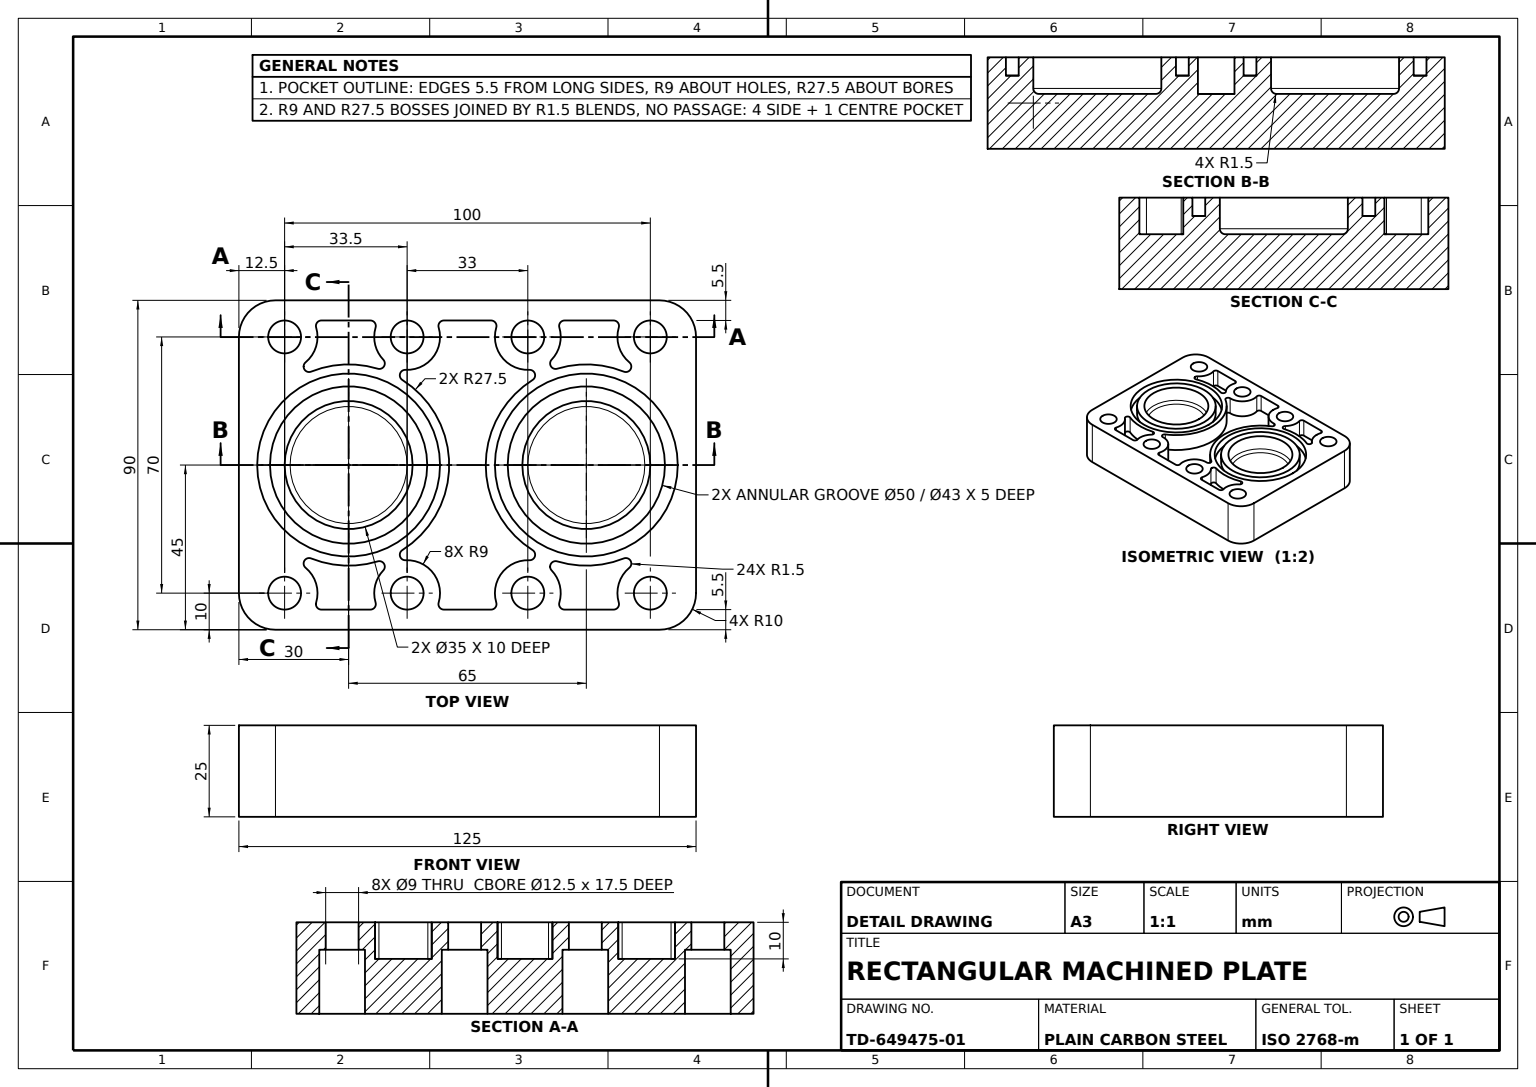
solid
v1 (-35,5,-22.75)
v2 (-35,5,-10.25)
e1 v1 v2 CIRCLE(AX(P(-35,5,-16.5),D(0,-1,0),D(0,0,-1)),6.25)
e2 v2 v1 CIRCLE(AX(P(-35,5,-16.5),D(0,-1,0),D(0,0,-1)),6.25)
v3 (-35,5,-21)
v4 (-35,5,-12)
e3 v3 v4 CIRCLE(AX(P(-35,5,-16.5),D(0,-1,0),D(0,0,-1)),4.5)
e4 v4 v3 CIRCLE(AX(P(-35,5,-16.5),D(0,-1,0),D(0,0,-1)),4.5)
face PLANE(AX(P(-30.5,5,-16.5),D(0,1,0),D(0,0,1))) rev [e1 e2] [-e3 -e4]
v5 (39.5,2.5,26.562306)
v6 (39.5,12.5,26.562306)
e5 v5 v6 LINE
v7 (39.5,2.5,39.937694)
e6 v7 v5 LINE
v8 (39.5,12.5,39.937694)
e7 v7 v8 LINE
e8 v8 v6 LINE
face PLANE(AX(P(39.5,2.5,26.562306),D(1,0,0),D(0,0,-1))) rev [-e5 -e6 e7 e8]
v9 (39.5,2.5,-6.437694)
v10 (39.5,12.5,-6.437694)
e9 v9 v10 LINE
v11 (37.571429,12.5,-7.875166)
e10 v10 v11 CIRCLE(AX(P(38,12.5,-6.437694),D(0,1,0),D(0,0,-1)),1.5)
v12 (37.571429,2.5,-7.875166)
e11 v12 v11 LINE
e12 v9 v12 CIRCLE(AX(P(38,2.5,-6.437694),D(0,1,0),D(0,0,-1)),1.5)
face CYL(AX(P(38,2.5,-6.437694),D(0,1,0),D(0,0,1)),1.5) rev [e9 e10 -e11 -e12]
v13 (0,12.5,7.5)
v14 (0,12.5,57.5)
e13 v13 v14 CIRCLE(AX(P(0,12.5,32.5),D(0,1,0),D(0,0,-1)),25)
v15 (0,7.5,57.5)
e14 v15 v14 LINE
v16 (0,7.5,7.5)
e15 v16 v15 CIRCLE(AX(P(0,7.5,32.5),D(0,1,0),D(0,0,-1)),25)
e16 v16 v13 LINE
face CYL(AX(P(0,7.5,32.5),D(0,1,0),D(0,0,1)),25) rev [e13 -e14 -e15 e16]
v17 (-35,5,43.75)
v18 (-35,5,56.25)
e17 v17 v18 CIRCLE(AX(P(-35,5,50),D(0,-1,0),D(0,0,-1)),6.25)
v19 (-35,-12.5,43.75)
e18 v17 v19 LINE
v20 (-35,-12.5,56.25)
e19 v19 v20 CIRCLE(AX(P(-35,-12.5,50),D(0,-1,0),D(0,0,-1)),6.25)
e20 v18 v20 LINE
face CYL(AX(P(-35,-12.5,50),D(0,-1,0),D(0,0,-1)),6.25) rev [-e17 e18 e19 -e20]
v21 (-28.792169,2.5,23.016351)
v22 (-35,2.5,25.5)
e21 v21 v22 CIRCLE(AX(P(-35,2.5,16.5),D(0,-1,0),D(0,0,1)),9)
v23 (-28.792169,12.5,23.016351)
e22 v21 v23 LINE
v24 (-35,12.5,25.5)
e23 v23 v24 CIRCLE(AX(P(-35,12.5,16.5),D(0,-1,0),D(0,0,1)),9)
e24 v22 v24 LINE
face CYL(AX(P(-35,2.5,16.5),D(0,1,0),D(0,0,1)),9) [-e21 e22 e23 -e24]
v25 (35,12.5,-21)
v26 (35,5,-21)
e25 v25 v26 LINE
v27 (35,5,-12)
e26 v26 v27 CIRCLE(AX(P(35,5,-16.5),D(0,-1,0),D(0,0,-1)),4.5)
v28 (35,12.5,-12)
e27 v28 v27 LINE
e28 v25 v28 CIRCLE(AX(P(35,12.5,-16.5),D(0,-1,0),D(0,0,-1)),4.5)
face CYL(AX(P(35,-12.5,-16.5),D(0,-1,0),D(0,0,-1)),4.5) rev [e25 e26 -e27 -e28]
v29 (35,5,22.75)
v30 (35,-12.5,22.75)
e29 v29 v30 LINE
v31 (35,-12.5,10.25)
e30 v30 v31 CIRCLE(AX(P(35,-12.5,16.5),D(0,-1,0),D(0,0,-1)),6.25)
v32 (35,5,10.25)
e31 v32 v31 LINE
e32 v29 v32 CIRCLE(AX(P(35,5,16.5),D(0,-1,0),D(0,0,-1)),6.25)
face CYL(AX(P(35,-12.5,16.5),D(0,-1,0),D(0,0,-1)),6.25) rev [e29 e30 -e31 -e32]
v33 (35,12.5,21)
v34 (35,5,21)
e33 v33 v34 LINE
v35 (35,12.5,12)
e34 v35 v33 CIRCLE(AX(P(35,12.5,16.5),D(0,-1,0),D(0,0,-1)),4.5)
v36 (35,5,12)
e35 v35 v36 LINE
e36 v36 v34 CIRCLE(AX(P(35,5,16.5),D(0,-1,0),D(0,0,-1)),4.5)
face CYL(AX(P(35,-12.5,16.5),D(0,-1,0),D(0,0,-1)),4.5) rev [-e33 -e34 e35 e36]
v37 (0,2.5,16.5)
v38 (0,2.5,48.5)
e37 v37 v38 CIRCLE(AX(P(0,2.5,32.5),D(0,1,0),D(0,0,1)),16)
e38 v38 v37 CIRCLE(AX(P(0,2.5,32.5),D(0,1,0),D(0,0,1)),16)
face PLANE(AX(P(0,2.5,32.5),D(0,1,0),D(0,0,1))) [e37 e38]
v39 (26.321796,2.5,-24.536768)
v40 (26.321796,12.5,-24.536768)
e39 v39 v40 LINE
v41 (27.75753,12.5,-22.602409)
e40 v40 v41 CIRCLE(AX(P(27.75753,12.5,-24.102409),D(0,1,0),D(0,0,-1)),1.5)
v42 (27.75753,2.5,-22.602409)
e41 v42 v41 LINE
e42 v39 v42 CIRCLE(AX(P(27.75753,2.5,-24.102409),D(0,1,0),D(0,0,-1)),1.5)
face CYL(AX(P(27.75753,2.5,-24.102409),D(0,1,0),D(0,0,1)),1.5) rev [e39 e40 -e41 -e42]
v43 (-23.244187,2.5,-17.804498)
v44 (-26.01033,2.5,-16.931078)
e43 v43 v44 CIRCLE(AX(P(-24.512051,2.5,-17.002925),D(0,1,0),D(0,0,1)),1.5)
v45 (-23.244187,12.5,-17.804498)
e44 v43 v45 LINE
v46 (-26.01033,12.5,-16.931078)
e45 v45 v46 CIRCLE(AX(P(-24.512051,12.5,-17.002925),D(0,1,0),D(0,0,1)),1.5)
e46 v44 v46 LINE
face CYL(AX(P(-24.512051,2.5,-17.002925),D(0,1,0),D(0,0,1)),1.5) rev [-e43 e44 e45 -e46]
v47 (35,12.5,-54.5)
v48 (35,5,-54.5)
e47 v47 v48 LINE
v49 (35,5,-45.5)
e48 v48 v49 CIRCLE(AX(P(35,5,-50),D(0,-1,0),D(0,0,-1)),4.5)
v50 (35,12.5,-45.5)
e49 v50 v49 LINE
e50 v47 v50 CIRCLE(AX(P(35,12.5,-50),D(0,-1,0),D(0,0,-1)),4.5)
face CYL(AX(P(35,-12.5,-50),D(0,-1,0),D(0,0,-1)),4.5) rev [e47 e48 -e49 -e50]
v51 (-35,12.5,-21)
e51 v51 v3 LINE
v52 (-35,12.5,-12)
e52 v52 v51 CIRCLE(AX(P(-35,12.5,-16.5),D(0,-1,0),D(0,0,-1)),4.5)
e53 v52 v4 LINE
face CYL(AX(P(-35,-12.5,-16.5),D(0,-1,0),D(0,0,-1)),4.5) rev [e4 -e51 -e52 e53]
v53 (0,4,-15)
v54 (0,4,-50)
e54 v53 v54 CIRCLE(AX(P(0,4,-32.5),D(0,-1,0),D(0,0,1)),17.5)
v55 (0,12.5,-50)
e55 v54 v55 LINE
v56 (0,12.5,-15)
e56 v55 v56 CIRCLE(AX(P(0,12.5,-32.5),D(0,1,0),D(0,0,1)),17.5)
e57 v53 v56 LINE
face CYL(AX(P(0,2.5,-32.5),D(0,1,0),D(0,0,1)),17.5) rev [e54 e55 e56 -e57]
v57 (37.571429,12.5,-41.375166)
v58 (35,12.5,-41)
e58 v57 v58 CIRCLE(AX(P(35,12.5,-50),D(0,-1,0),D(0,0,-1)),9)
v59 (35,2.5,-41)
e59 v59 v58 LINE
v60 (37.571429,2.5,-41.375166)
e60 v60 v59 CIRCLE(AX(P(35,2.5,-50),D(0,-1,0),D(0,0,-1)),9)
e61 v60 v57 LINE
face CYL(AX(P(35,2.5,-50),D(0,1,0),D(0,0,1)),9) [e58 -e59 -e60 e61]
e62 v51 v52 CIRCLE(AX(P(-35,12.5,-16.5),D(0,-1,0),D(0,0,-1)),4.5)
face CYL(AX(P(-35,-12.5,-16.5),D(0,-1,0),D(0,0,-1)),4.5) rev [e51 e3 -e53 -e62]
v61 (35,5,-10.25)
v62 (35,5,-22.75)
e63 v61 v62 CIRCLE(AX(P(35,5,-16.5),D(0,-1,0),D(0,0,-1)),6.25)
e64 v62 v61 CIRCLE(AX(P(35,5,-16.5),D(0,-1,0),D(0,0,-1)),6.25)
e65 v27 v26 CIRCLE(AX(P(35,5,-16.5),D(0,-1,0),D(0,0,-1)),4.5)
face PLANE(AX(P(39.5,5,-16.5),D(0,1,0),D(0,0,1))) rev [e63 e64] [-e26 -e65]
v63 (35,5,-56.25)
v64 (35,5,-43.75)
e66 v63 v64 CIRCLE(AX(P(35,5,-50),D(0,-1,0),D(0,0,-1)),6.25)
e67 v64 v63 CIRCLE(AX(P(35,5,-50),D(0,-1,0),D(0,0,-1)),6.25)
e68 v49 v48 CIRCLE(AX(P(35,5,-50),D(0,-1,0),D(0,0,-1)),4.5)
face PLANE(AX(P(39.5,5,-50),D(0,1,0),D(0,0,1))) rev [e66 e67] [-e48 -e68]
v65 (-37.571429,2.5,25.124834)
v66 (-39.5,2.5,26.562306)
e69 v65 v66 CIRCLE(AX(P(-38,2.5,26.562306),D(0,1,0),D(0,0,1)),1.5)
v67 (-37.571429,12.5,25.124834)
e70 v65 v67 LINE
v68 (-39.5,12.5,26.562306)
e71 v67 v68 CIRCLE(AX(P(-38,12.5,26.562306),D(0,1,0),D(0,0,1)),1.5)
e72 v66 v68 LINE
face CYL(AX(P(-38,2.5,26.562306),D(0,1,0),D(0,0,1)),1.5) rev [-e69 e70 e71 -e72]
v69 (38,2.5,41.437694)
v70 (38,12.5,41.437694)
e73 v69 v70 LINE
e74 v70 v8 CIRCLE(AX(P(38,12.5,39.937694),D(0,1,0),D(0,0,1)),1.5)
e75 v69 v7 CIRCLE(AX(P(38,2.5,39.937694),D(0,1,0),D(0,0,1)),1.5)
face CYL(AX(P(38,2.5,39.937694),D(0,1,0),D(0,0,1)),1.5) rev [e73 e74 -e7 -e75]
v71 (35,5,45.5)
v72 (35,5,54.5)
e76 v71 v72 CIRCLE(AX(P(35,5,50),D(0,-1,0),D(0,0,-1)),4.5)
e77 v72 v71 CIRCLE(AX(P(35,5,50),D(0,-1,0),D(0,0,-1)),4.5)
v73 (35,5,56.25)
v74 (35,5,43.75)
e78 v73 v74 CIRCLE(AX(P(35,5,50),D(0,-1,0),D(0,0,-1)),6.25)
e79 v74 v73 CIRCLE(AX(P(35,5,50),D(0,-1,0),D(0,0,-1)),6.25)
face PLANE(AX(P(39.5,5,50),D(0,1,0),D(0,0,1))) rev [-e76 -e77] [e78 e79]
v75 (39.5,2.5,-26.562306)
v76 (39.5,12.5,-26.562306)
e80 v75 v76 LINE
v77 (38,2.5,-25.062306)
e81 v77 v75 CIRCLE(AX(P(38,2.5,-26.562306),D(0,1,0),D(0,0,1)),1.5)
v78 (38,12.5,-25.062306)
e82 v77 v78 LINE
e83 v78 v76 CIRCLE(AX(P(38,12.5,-26.562306),D(0,1,0),D(0,0,1)),1.5)
face CYL(AX(P(38,2.5,-26.562306),D(0,1,0),D(0,0,1)),1.5) rev [-e80 -e81 e82 e83]
v79 (26.01033,2.5,16.931078)
v80 (26.01033,12.5,16.931078)
e84 v79 v80 LINE
v81 (37.571429,12.5,7.875166)
e85 v80 v81 CIRCLE(AX(P(35,12.5,16.5),D(0,-1,0),D(0,0,-1)),9)
v82 (37.571429,2.5,7.875166)
e86 v82 v81 LINE
e87 v79 v82 CIRCLE(AX(P(35,2.5,16.5),D(0,-1,0),D(0,0,-1)),9)
face CYL(AX(P(35,2.5,16.5),D(0,1,0),D(0,0,1)),9) [e84 e85 -e86 -e87]
v83 (0,4,15)
e88 v37 v83 CIRCLE(AX(P(0,4,16.5),D(1,0,0),D(0,0,-1)),1.5)
v84 (0,4,50)
e89 v84 v83 CIRCLE(AX(P(0,4,32.5),D(0,-1,0),D(0,0,1)),17.5)
e90 v38 v84 CIRCLE(AX(P(0,4,48.5),D(-1,0,0),D(0,0,1)),1.5)
face TORUS(AX(P(0,4,32.5),D(0,1,0),D(0,0,1)),16,1.5) rev [e88 -e89 -e90 -e37]
v85 (38,12.5,7.937694)
v86 (39.5,12.5,6.437694)
e91 v85 v86 CIRCLE(AX(P(38,12.5,6.437694),D(0,1,0),D(0,0,1)),1.5)
v87 (39.5,2.5,6.437694)
e92 v87 v86 LINE
v88 (38,2.5,7.937694)
e93 v88 v87 CIRCLE(AX(P(38,2.5,6.437694),D(0,1,0),D(0,0,1)),1.5)
e94 v88 v85 LINE
face CYL(AX(P(38,2.5,6.437694),D(0,1,0),D(0,0,1)),1.5) rev [e91 -e92 -e93 e94]
v89 (35,2.5,-7.5)
v90 (35,12.5,-7.5)
e95 v89 v90 LINE
v91 (26.01033,12.5,-16.931078)
e96 v90 v91 CIRCLE(AX(P(35,12.5,-16.5),D(0,-1,0),D(0,0,-1)),9)
v92 (26.01033,2.5,-16.931078)
e97 v92 v91 LINE
e98 v89 v92 CIRCLE(AX(P(35,2.5,-16.5),D(0,-1,0),D(0,0,-1)),9)
face CYL(AX(P(35,2.5,-16.5),D(0,1,0),D(0,0,1)),9) [e95 e96 -e97 -e98]
v93 (-37.571429,12.5,41.375166)
v94 (-28.067872,12.5,44.260174)
e99 v93 v94 CIRCLE(AX(P(-35,12.5,50),D(0,-1,0),D(0,0,1)),9)
v95 (-28.067872,2.5,44.260174)
e100 v95 v94 LINE
v96 (-37.571429,2.5,41.375166)
e101 v96 v95 CIRCLE(AX(P(-35,2.5,50),D(0,-1,0),D(0,0,1)),9)
e102 v96 v93 LINE
face CYL(AX(P(-35,2.5,50),D(0,1,0),D(0,0,1)),9) [e99 -e100 -e101 e102]
v97 (0,2.5,-16.5)
v98 (0,2.5,-48.5)
e103 v97 v98 CIRCLE(AX(P(0,2.5,-32.5),D(0,1,0),D(0,0,1)),16)
e104 v98 v97 CIRCLE(AX(P(0,2.5,-32.5),D(0,1,0),D(0,0,1)),16)
face PLANE(AX(P(0,2.5,-32.5),D(0,1,0),D(0,0,1))) [e103 e104]
v99 (-24.512051,2.5,18.502925)
v100 (-24.512051,12.5,18.502925)
e105 v99 v100 LINE
v101 (-26.01033,2.5,16.931078)
e106 v101 v99 CIRCLE(AX(P(-24.512051,2.5,17.002925),D(0,1,0),D(0,0,1)),1.5)
v102 (-26.01033,12.5,16.931078)
e107 v101 v102 LINE
e108 v102 v100 CIRCLE(AX(P(-24.512051,12.5,17.002925),D(0,1,0),D(0,0,1)),1.5)
face CYL(AX(P(-24.512051,2.5,17.002925),D(0,1,0),D(0,0,1)),1.5) rev [-e105 -e106 e107 e108]
v103 (0,7.5,11)
v104 (0,12.5,11)
e109 v103 v104 LINE
v105 (0,12.5,54)
e110 v105 v104 CIRCLE(AX(P(0,12.5,32.5),D(0,1,0),D(0,0,-1)),21.5)
v106 (0,7.5,54)
e111 v106 v105 LINE
e112 v106 v103 CIRCLE(AX(P(0,7.5,32.5),D(0,1,0),D(0,0,-1)),21.5)
face CYL(AX(P(0,7.5,32.5),D(0,1,0),D(0,0,1)),21.5) [e109 -e110 -e111 e112]
v107 (-35,12.5,54.5)
v108 (-35,5,54.5)
e113 v107 v108 LINE
v109 (-35,5,45.5)
e114 v108 v109 CIRCLE(AX(P(-35,5,50),D(0,-1,0),D(0,0,-1)),4.5)
v110 (-35,12.5,45.5)
e115 v110 v109 LINE
e116 v107 v110 CIRCLE(AX(P(-35,12.5,50),D(0,-1,0),D(0,0,-1)),4.5)
face CYL(AX(P(-35,-12.5,50),D(0,-1,0),D(0,0,-1)),4.5) rev [e113 e114 -e115 -e116]
v111 (-38,12.5,41.437694)
e117 v111 v93 CIRCLE(AX(P(-38,12.5,39.937694),D(0,1,0),D(0,0,-1)),1.5)
v112 (-38,2.5,41.437694)
e118 v112 v96 CIRCLE(AX(P(-38,2.5,39.937694),D(0,1,0),D(0,0,-1)),1.5)
e119 v112 v111 LINE
face CYL(AX(P(-38,2.5,39.937694),D(0,1,0),D(0,0,1)),1.5) rev [e117 -e102 -e118 e119]
v113 (28.067872,12.5,44.260174)
v114 (37.571429,12.5,41.375166)
e120 v113 v114 CIRCLE(AX(P(35,12.5,50),D(0,-1,0),D(0,0,-1)),9)
v115 (37.571429,2.5,41.375166)
e121 v115 v114 LINE
v116 (28.067872,2.5,44.260174)
e122 v116 v115 CIRCLE(AX(P(35,2.5,50),D(0,-1,0),D(0,0,-1)),9)
e123 v116 v113 LINE
face CYL(AX(P(35,2.5,50),D(0,1,0),D(0,0,1)),9) [e120 -e121 -e122 e123]
v117 (-23.244187,2.5,17.804498)
v118 (-23.244187,12.5,17.804498)
e124 v117 v118 LINE
e125 v99 v117 CIRCLE(AX(P(-24.512051,2.5,17.002925),D(0,1,0),D(0,0,1)),1.5)
e126 v100 v118 CIRCLE(AX(P(-24.512051,12.5,17.002925),D(0,1,0),D(0,0,1)),1.5)
face CYL(AX(P(-24.512051,2.5,17.002925),D(0,1,0),D(0,0,1)),1.5) rev [-e124 -e125 e105 e126]
v119 (-35,5,-43.75)
v120 (-35,5,-56.25)
e127 v119 v120 CIRCLE(AX(P(-35,5,-50),D(0,-1,0),D(0,0,-1)),6.25)
v121 (-35,-12.5,-43.75)
e128 v119 v121 LINE
v122 (-35,-12.5,-56.25)
e129 v121 v122 CIRCLE(AX(P(-35,-12.5,-50),D(0,-1,0),D(0,0,-1)),6.25)
e130 v120 v122 LINE
face CYL(AX(P(-35,-12.5,-50),D(0,-1,0),D(0,0,-1)),6.25) rev [-e127 e128 e129 -e130]
v123 (24.512051,2.5,18.502925)
e131 v123 v79 CIRCLE(AX(P(24.512051,2.5,17.002925),D(0,1,0),D(0,0,-1)),1.5)
v124 (24.512051,12.5,18.502925)
e132 v123 v124 LINE
e133 v124 v80 CIRCLE(AX(P(24.512051,12.5,17.002925),D(0,1,0),D(0,0,-1)),1.5)
face CYL(AX(P(24.512051,2.5,17.002925),D(0,1,0),D(0,0,1)),1.5) rev [-e84 -e131 e132 e133]
e134 v109 v108 CIRCLE(AX(P(-35,5,50),D(0,-1,0),D(0,0,-1)),4.5)
e135 v110 v107 CIRCLE(AX(P(-35,12.5,50),D(0,-1,0),D(0,0,-1)),4.5)
face CYL(AX(P(-35,-12.5,50),D(0,-1,0),D(0,0,-1)),4.5) rev [e134 -e113 -e135 e115]
v125 (0,12.5,50)
e136 v84 v125 LINE
v126 (0,12.5,15)
e137 v83 v126 LINE
e138 v126 v125 CIRCLE(AX(P(0,12.5,32.5),D(0,1,0),D(0,0,1)),17.5)
face CYL(AX(P(0,2.5,32.5),D(0,1,0),D(0,0,1)),17.5) rev [-e136 e89 e137 e138]
v127 (0,7.5,-57.5)
v128 (0,7.5,-7.5)
e139 v127 v128 CIRCLE(AX(P(0,7.5,-32.5),D(0,1,0),D(0,0,1)),25)
e140 v128 v127 CIRCLE(AX(P(0,7.5,-32.5),D(0,1,0),D(0,0,1)),25)
v129 (0,7.5,-54)
v130 (0,7.5,-11)
e141 v129 v130 CIRCLE(AX(P(0,7.5,-32.5),D(0,1,0),D(0,0,1)),21.5)
e142 v130 v129 CIRCLE(AX(P(0,7.5,-32.5),D(0,1,0),D(0,0,1)),21.5)
face PLANE(AX(P(0,7.5,-32.5),D(0,1,0),D(0,0,1))) [e139 e140] [-e141 -e142]
v131 (23.244187,2.5,17.804498)
e143 v131 v123 CIRCLE(AX(P(24.512051,2.5,17.002925),D(0,1,0),D(0,0,-1)),1.5)
v132 (23.244187,12.5,17.804498)
e144 v131 v132 LINE
e145 v132 v124 CIRCLE(AX(P(24.512051,12.5,17.002925),D(0,1,0),D(0,0,-1)),1.5)
face CYL(AX(P(24.512051,2.5,17.002925),D(0,1,0),D(0,0,1)),1.5) rev [-e143 e144 e145 -e132]
v133 (-38,2.5,-25.062306)
v134 (-38,12.5,-25.062306)
e146 v133 v134 LINE
v135 (-37.571429,12.5,-25.124834)
e147 v134 v135 CIRCLE(AX(P(-38,12.5,-26.562306),D(0,1,0),D(0,0,-1)),1.5)
v136 (-37.571429,2.5,-25.124834)
e148 v136 v135 LINE
e149 v133 v136 CIRCLE(AX(P(-38,2.5,-26.562306),D(0,1,0),D(0,0,-1)),1.5)
face CYL(AX(P(-38,2.5,-26.562306),D(0,1,0),D(0,0,1)),1.5) rev [e146 e147 -e148 -e149]
v137 (35,-12.5,-43.75)
v138 (35,-12.5,-56.25)
e150 v137 v138 CIRCLE(AX(P(35,-12.5,-50),D(0,-1,0),D(0,0,-1)),6.25)
e151 v63 v138 LINE
e152 v64 v137 LINE
face CYL(AX(P(35,-12.5,-50),D(0,-1,0),D(0,0,-1)),6.25) rev [e150 -e151 -e67 e152]
v139 (-45,-12.5,52.5)
v140 (-45,-12.5,-52.5)
e153 v139 v140 LINE
v141 (-45,12.5,52.5)
e154 v139 v141 LINE
v142 (-45,12.5,-52.5)
e155 v142 v141 LINE
e156 v142 v140 LINE
face PLANE(AX(P(-45,0,0),D(1,0,0),D(0,0,-1))) rev [-e153 e154 -e155 e156]
e157 v83 v84 CIRCLE(AX(P(0,4,32.5),D(0,-1,0),D(0,0,1)),17.5)
face TORUS(AX(P(0,4,32.5),D(0,1,0),D(0,0,1)),16,1.5) rev [-e38 e90 -e157 -e88]
e158 v138 v137 CIRCLE(AX(P(35,-12.5,-50),D(0,-1,0),D(0,0,-1)),6.25)
face CYL(AX(P(35,-12.5,-50),D(0,-1,0),D(0,0,-1)),6.25) rev [-e66 e151 e158 -e152]
v143 (35,12.5,45.5)
e159 v143 v71 LINE
v144 (35,12.5,54.5)
e160 v144 v143 CIRCLE(AX(P(35,12.5,50),D(0,-1,0),D(0,0,-1)),4.5)
e161 v144 v72 LINE
face CYL(AX(P(35,-12.5,50),D(0,-1,0),D(0,0,-1)),4.5) rev [-e159 -e160 e161 e77]
v145 (-35,-12.5,-10.25)
e162 v2 v145 LINE
v146 (-35,-12.5,-22.75)
e163 v1 v146 LINE
e164 v146 v145 CIRCLE(AX(P(-35,-12.5,-16.5),D(0,-1,0),D(0,0,-1)),6.25)
face CYL(AX(P(-35,-12.5,-16.5),D(0,-1,0),D(0,0,-1)),6.25) rev [-e162 -e1 e163 e164]
v147 (-28.067872,2.5,-44.260174)
v148 (-28.067872,12.5,-44.260174)
e165 v147 v148 LINE
v149 (-35,12.5,-41)
e166 v148 v149 CIRCLE(AX(P(-35,12.5,-50),D(0,-1,0),D(0,0,1)),9)
v150 (-35,2.5,-41)
e167 v150 v149 LINE
e168 v147 v150 CIRCLE(AX(P(-35,2.5,-50),D(0,-1,0),D(0,0,1)),9)
face CYL(AX(P(-35,2.5,-50),D(0,1,0),D(0,0,1)),9) [e165 e166 -e167 -e168]
v151 (-25.520491,2.5,42.744732)
v152 (-25.520491,12.5,42.744732)
e169 v151 v152 LINE
v153 (-26.912518,2.5,44.803536)
e170 v153 v151 CIRCLE(AX(P(-26.912518,2.5,43.303536),D(0,1,0),D(0,0,1)),1.5)
v154 (-26.912518,12.5,44.803536)
e171 v153 v154 LINE
e172 v154 v152 CIRCLE(AX(P(-26.912518,12.5,43.303536),D(0,1,0),D(0,0,1)),1.5)
face CYL(AX(P(-26.912518,2.5,43.303536),D(0,1,0),D(0,0,1)),1.5) rev [-e169 -e170 e171 e172]
e173 v33 v35 CIRCLE(AX(P(35,12.5,16.5),D(0,-1,0),D(0,0,-1)),4.5)
e174 v34 v36 CIRCLE(AX(P(35,5,16.5),D(0,-1,0),D(0,0,-1)),4.5)
face CYL(AX(P(35,-12.5,16.5),D(0,-1,0),D(0,0,-1)),4.5) rev [-e35 -e173 e33 e174]
v155 (-35,12.5,62.5)
v156 (-35,-12.5,62.5)
e175 v155 v156 LINE
e176 v141 v155 CIRCLE(AX(P(-35,12.5,52.5),D(0,1,0),D(0,0,-1)),10)
e177 v156 v139 CIRCLE(AX(P(-35,-12.5,52.5),D(0,-1,0),D(0,0,1)),10)
face CYL(AX(P(-35,12.5,52.5),D(0,-1,0),D(0,0,-1)),10) [-e175 -e176 -e154 -e177]
e178 v20 v19 CIRCLE(AX(P(-35,-12.5,50),D(0,-1,0),D(0,0,-1)),6.25)
e179 v18 v17 CIRCLE(AX(P(-35,5,50),D(0,-1,0),D(0,0,-1)),6.25)
face CYL(AX(P(-35,-12.5,50),D(0,-1,0),D(0,0,-1)),6.25) rev [e20 e178 -e18 -e179]
v157 (39.5,12.5,-39.937694)
e180 v157 v57 CIRCLE(AX(P(38,12.5,-39.937694),D(0,1,0),D(0,0,-1)),1.5)
v158 (39.5,2.5,-39.937694)
e181 v158 v60 CIRCLE(AX(P(38,2.5,-39.937694),D(0,1,0),D(0,0,-1)),1.5)
e182 v158 v157 LINE
face CYL(AX(P(38,2.5,-39.937694),D(0,1,0),D(0,0,1)),1.5) rev [e180 -e61 -e181 e182]
v159 (-35,12.5,21)
v160 (-35,12.5,12)
e183 v159 v160 CIRCLE(AX(P(-35,12.5,16.5),D(0,-1,0),D(0,0,-1)),4.5)
v161 (-35,5,21)
e184 v159 v161 LINE
v162 (-35,5,12)
e185 v161 v162 CIRCLE(AX(P(-35,5,16.5),D(0,-1,0),D(0,0,-1)),4.5)
e186 v160 v162 LINE
face CYL(AX(P(-35,-12.5,16.5),D(0,-1,0),D(0,0,-1)),4.5) rev [-e183 e184 e185 -e186]
e187 v76 v157 LINE
e188 v75 v158 LINE
face PLANE(AX(P(39.5,2.5,-39.937694),D(1,0,0),D(0,0,-1))) rev [e187 -e182 -e188 e80]
v163 (37.571429,2.5,-25.124834)
e189 v163 v77 CIRCLE(AX(P(38,2.5,-26.562306),D(0,1,0),D(0,0,1)),1.5)
v164 (28.067872,2.5,-44.260174)
e190 v59 v164 CIRCLE(AX(P(35,2.5,-50),D(0,-1,0),D(0,0,-1)),9)
v165 (25.520491,2.5,-42.744732)
e191 v164 v165 CIRCLE(AX(P(26.912518,2.5,-43.303536),D(0,1,0),D(0,0,-1)),1.5)
e192 v165 v39 CIRCLE(AX(P(0,2.5,-32.5),D(0,-1,0),D(0,0,1)),27.5)
v166 (28.792169,2.5,-23.016351)
e193 v42 v166 CIRCLE(AX(P(27.75753,2.5,-24.102409),D(0,1,0),D(0,0,-1)),1.5)
e194 v166 v163 CIRCLE(AX(P(35,2.5,-16.5),D(0,-1,0),D(0,0,-1)),9)
face PLANE(AX(P(35,2.5,-50),D(0,-1,0),D(0,0,-1))) rev [e189 e81 e188 e181 e60 e190 e191 e192 e42 e193 e194]
face PLANE(AX(P(-30.5,5,50),D(0,1,0),D(0,0,1))) rev [-e114 -e134] [e17 e179]
v167 (37.571429,2.5,25.124834)
e195 v5 v167 CIRCLE(AX(P(38,2.5,26.562306),D(0,1,0),D(0,0,-1)),1.5)
v168 (35,2.5,25.5)
e196 v167 v168 CIRCLE(AX(P(35,2.5,16.5),D(0,-1,0),D(0,0,-1)),9)
v169 (28.792169,2.5,23.016351)
e197 v168 v169 CIRCLE(AX(P(35,2.5,16.5),D(0,-1,0),D(0,0,-1)),9)
v170 (26.321796,2.5,24.536768)
e198 v169 v170 CIRCLE(AX(P(27.75753,2.5,24.102409),D(0,1,0),D(0,0,-1)),1.5)
v171 (25.520491,2.5,42.744732)
e199 v170 v171 CIRCLE(AX(P(0,2.5,32.5),D(0,-1,0),D(0,0,1)),27.5)
v172 (26.912518,2.5,44.803536)
e200 v171 v172 CIRCLE(AX(P(26.912518,2.5,43.303536),D(0,1,0),D(0,0,-1)),1.5)
e201 v172 v116 CIRCLE(AX(P(26.912518,2.5,43.303536),D(0,1,0),D(0,0,-1)),1.5)
e202 v115 v69 CIRCLE(AX(P(38,2.5,39.937694),D(0,1,0),D(0,0,1)),1.5)
face PLANE(AX(P(35,2.5,50),D(0,-1,0),D(0,0,-1))) rev [e6 e195 e196 e197 e198 e199 e200 e201 e122 e202 e75]
v173 (25.520491,12.5,-42.744732)
e203 v165 v173 LINE
e204 v173 v40 CIRCLE(AX(P(0,12.5,-32.5),D(0,-1,0),D(0,0,1)),27.5)
face CYL(AX(P(0,2.5,-32.5),D(0,1,0),D(0,0,1)),27.5) [-e39 -e192 e203 e204]
v174 (28.792169,12.5,-23.016351)
e205 v41 v174 CIRCLE(AX(P(27.75753,12.5,-24.102409),D(0,1,0),D(0,0,-1)),1.5)
e206 v166 v174 LINE
face CYL(AX(P(27.75753,2.5,-24.102409),D(0,1,0),D(0,0,1)),1.5) rev [e205 -e206 -e193 e41]
v175 (0,2.5,-5)
e207 v175 v43 CIRCLE(AX(P(0,2.5,-32.5),D(0,-1,0),D(0,0,1)),27.5)
v176 (0,12.5,-5)
e208 v175 v176 LINE
e209 v176 v45 CIRCLE(AX(P(0,12.5,-32.5),D(0,-1,0),D(0,0,1)),27.5)
face CYL(AX(P(0,2.5,-32.5),D(0,1,0),D(0,0,1)),27.5) [-e44 -e207 e208 e209]
v177 (0,12.5,-7.5)
e210 v128 v177 LINE
v178 (0,12.5,-57.5)
e211 v127 v178 LINE
e212 v178 v177 CIRCLE(AX(P(0,12.5,-32.5),D(0,1,0),D(0,0,1)),25)
face CYL(AX(P(0,7.5,-32.5),D(0,1,0),D(0,0,1)),25) rev [-e210 -e139 e211 e212]
v179 (35,-12.5,56.25)
e213 v73 v179 LINE
v180 (35,-12.5,43.75)
e214 v179 v180 CIRCLE(AX(P(35,-12.5,50),D(0,-1,0),D(0,0,-1)),6.25)
e215 v74 v180 LINE
face CYL(AX(P(35,-12.5,50),D(0,-1,0),D(0,0,-1)),6.25) rev [-e78 e213 e214 -e215]
v181 (25.520491,12.5,42.744732)
e216 v171 v181 LINE
v182 (26.912518,12.5,44.803536)
e217 v181 v182 CIRCLE(AX(P(26.912518,12.5,43.303536),D(0,1,0),D(0,0,-1)),1.5)
e218 v172 v182 LINE
face CYL(AX(P(26.912518,2.5,43.303536),D(0,1,0),D(0,0,1)),1.5) rev [-e200 e216 e217 -e218]
v183 (-26.321796,2.5,-24.536768)
v184 (-25.520491,2.5,-42.744732)
e219 v183 v184 CIRCLE(AX(P(0,2.5,-32.5),D(0,-1,0),D(0,0,1)),27.5)
v185 (-26.321796,12.5,-24.536768)
e220 v183 v185 LINE
v186 (-25.520491,12.5,-42.744732)
e221 v185 v186 CIRCLE(AX(P(0,12.5,-32.5),D(0,-1,0),D(0,0,1)),27.5)
e222 v184 v186 LINE
face CYL(AX(P(0,2.5,-32.5),D(0,1,0),D(0,0,1)),27.5) [-e219 e220 e221 -e222]
e223 v125 v126 CIRCLE(AX(P(0,12.5,32.5),D(0,1,0),D(0,0,1)),17.5)
e224 v104 v105 CIRCLE(AX(P(0,12.5,32.5),D(0,1,0),D(0,0,-1)),21.5)
face PLANE(AX(P(45,12.5,62.5),D(0,-1,0),D(0,0,-1))) rev [-e138 -e223] [e224 e110]
v187 (-37.571429,2.5,-41.375166)
e225 v150 v187 CIRCLE(AX(P(-35,2.5,-50),D(0,-1,0),D(0,0,1)),9)
v188 (-37.571429,12.5,-41.375166)
e226 v149 v188 CIRCLE(AX(P(-35,12.5,-50),D(0,-1,0),D(0,0,1)),9)
e227 v187 v188 LINE
face CYL(AX(P(-35,2.5,-50),D(0,1,0),D(0,0,1)),9) [-e225 e167 e226 -e227]
v189 (-37.571429,2.5,7.875166)
e228 v189 v101 CIRCLE(AX(P(-35,2.5,16.5),D(0,-1,0),D(0,0,1)),9)
v190 (-37.571429,12.5,7.875166)
e229 v189 v190 LINE
e230 v190 v102 CIRCLE(AX(P(-35,12.5,16.5),D(0,-1,0),D(0,0,1)),9)
face CYL(AX(P(-35,2.5,16.5),D(0,1,0),D(0,0,1)),9) [-e228 e229 e230 -e107]
v191 (-39.5,2.5,-39.937694)
v192 (-39.5,2.5,-26.562306)
e231 v191 v192 LINE
v193 (-39.5,12.5,-39.937694)
e232 v191 v193 LINE
v194 (-39.5,12.5,-26.562306)
e233 v193 v194 LINE
e234 v192 v194 LINE
face PLANE(AX(P(-39.5,2.5,-39.937694),D(-1,0,0),D(0,0,1))) rev [-e231 e232 e233 -e234]
e235 v87 v9 LINE
e236 v86 v10 LINE
face PLANE(AX(P(39.5,2.5,-6.437694),D(1,0,0),D(0,0,-1))) rev [-e235 e92 e236 -e9]
v195 (35,12.5,25.5)
e237 v168 v195 LINE
v196 (28.792169,12.5,23.016351)
e238 v195 v196 CIRCLE(AX(P(35,12.5,16.5),D(0,-1,0),D(0,0,-1)),9)
e239 v169 v196 LINE
face CYL(AX(P(35,2.5,16.5),D(0,1,0),D(0,0,1)),9) [e237 e238 -e239 -e197]
v197 (-35,2.5,-7.5)
v198 (-35,12.5,-7.5)
e240 v197 v198 LINE
e241 v44 v197 CIRCLE(AX(P(-35,2.5,-16.5),D(0,-1,0),D(0,0,1)),9)
e242 v46 v198 CIRCLE(AX(P(-35,12.5,-16.5),D(0,-1,0),D(0,0,1)),9)
face CYL(AX(P(-35,2.5,-16.5),D(0,1,0),D(0,0,1)),9) [-e240 -e241 e46 e242]
e243 v194 v134 CIRCLE(AX(P(-38,12.5,-26.562306),D(0,1,0),D(0,0,-1)),1.5)
e244 v192 v133 CIRCLE(AX(P(-38,2.5,-26.562306),D(0,1,0),D(0,0,-1)),1.5)
face CYL(AX(P(-38,2.5,-26.562306),D(0,1,0),D(0,0,1)),1.5) rev [e234 e243 -e146 -e244]
e245 v22 v65 CIRCLE(AX(P(-35,2.5,16.5),D(0,-1,0),D(0,0,1)),9)
e246 v24 v67 CIRCLE(AX(P(-35,12.5,16.5),D(0,-1,0),D(0,0,1)),9)
face CYL(AX(P(-35,2.5,16.5),D(0,1,0),D(0,0,1)),9) [-e70 -e245 e24 e246]
v199 (-37.571429,2.5,-7.875166)
v200 (-37.571429,12.5,-7.875166)
e247 v199 v200 LINE
e248 v197 v199 CIRCLE(AX(P(-35,2.5,-16.5),D(0,-1,0),D(0,0,1)),9)
e249 v198 v200 CIRCLE(AX(P(-35,12.5,-16.5),D(0,-1,0),D(0,0,1)),9)
face CYL(AX(P(-35,2.5,-16.5),D(0,1,0),D(0,0,1)),9) [-e247 -e248 e240 e249]
e250 v162 v161 CIRCLE(AX(P(-35,5,16.5),D(0,-1,0),D(0,0,-1)),4.5)
e251 v160 v159 CIRCLE(AX(P(-35,12.5,16.5),D(0,-1,0),D(0,0,-1)),4.5)
face CYL(AX(P(-35,-12.5,16.5),D(0,-1,0),D(0,0,-1)),4.5) rev [e250 -e184 -e251 e186]
v201 (-39.5,12.5,39.937694)
e252 v68 v201 LINE
v202 (-39.5,2.5,39.937694)
e253 v202 v201 LINE
e254 v66 v202 LINE
face PLANE(AX(P(-39.5,2.5,26.562306),D(-1,0,0),D(0,0,1))) rev [e252 -e253 -e254 e72]
e255 v81 v85 CIRCLE(AX(P(38,12.5,6.437694),D(0,1,0),D(0,0,1)),1.5)
e256 v82 v88 CIRCLE(AX(P(38,2.5,6.437694),D(0,1,0),D(0,0,1)),1.5)
face CYL(AX(P(38,2.5,6.437694),D(0,1,0),D(0,0,1)),1.5) rev [e86 e255 -e94 -e256]
e257 v32 v29 CIRCLE(AX(P(35,5,16.5),D(0,-1,0),D(0,0,-1)),6.25)
face PLANE(AX(P(39.5,5,16.5),D(0,1,0),D(0,0,1))) rev [-e36 -e174] [e32 e257]
v203 (-35,5,22.75)
v204 (-35,-12.5,22.75)
e258 v203 v204 LINE
v205 (-35,-12.5,10.25)
e259 v204 v205 CIRCLE(AX(P(-35,-12.5,16.5),D(0,-1,0),D(0,0,-1)),6.25)
v206 (-35,5,10.25)
e260 v206 v205 LINE
e261 v203 v206 CIRCLE(AX(P(-35,5,16.5),D(0,-1,0),D(0,0,-1)),6.25)
face CYL(AX(P(-35,-12.5,16.5),D(0,-1,0),D(0,0,-1)),6.25) rev [e258 e259 -e260 -e261]
v207 (35,12.5,-62.5)
v208 (35,-12.5,-62.5)
e262 v207 v208 LINE
v209 (-35,-12.5,-62.5)
e263 v208 v209 LINE
v210 (-35,12.5,-62.5)
e264 v209 v210 LINE
e265 v207 v210 LINE
face PLANE(AX(P(45,12.5,-62.5),D(0,0,1),D(1,0,0))) rev [e262 e263 e264 -e265]
v211 (-39.5,2.5,6.437694)
v212 (-39.5,12.5,6.437694)
e266 v211 v212 LINE
v213 (-38,12.5,7.937694)
e267 v212 v213 CIRCLE(AX(P(-38,12.5,6.437694),D(0,1,0),D(0,0,-1)),1.5)
v214 (-38,2.5,7.937694)
e268 v214 v213 LINE
e269 v211 v214 CIRCLE(AX(P(-38,2.5,6.437694),D(0,1,0),D(0,0,-1)),1.5)
face CYL(AX(P(-38,2.5,6.437694),D(0,1,0),D(0,0,1)),1.5) rev [e266 e267 -e268 -e269]
v215 (28.067872,12.5,-44.260174)
e270 v164 v215 LINE
e271 v215 v173 CIRCLE(AX(P(26.912518,12.5,-43.303536),D(0,1,0),D(0,0,-1)),1.5)
face CYL(AX(P(26.912518,2.5,-43.303536),D(0,1,0),D(0,0,1)),1.5) rev [-e203 -e191 e270 e271]
e272 v140 v209 CIRCLE(AX(P(-35,-12.5,-52.5),D(0,-1,0),D(0,0,1)),10)
e273 v210 v142 CIRCLE(AX(P(-35,12.5,-52.5),D(0,1,0),D(0,0,-1)),10)
face CYL(AX(P(-35,12.5,-52.5),D(0,1,0),D(0,0,1)),10) [-e272 -e156 -e273 -e264]
e274 v117 v131 CIRCLE(AX(P(0,2.5,32.5),D(0,-1,0),D(0,0,1)),27.5)
e275 v12 v89 CIRCLE(AX(P(35,2.5,-16.5),D(0,-1,0),D(0,0,-1)),9)
v216 (23.244187,2.5,-17.804498)
e276 v92 v216 CIRCLE(AX(P(24.512051,2.5,-17.002925),D(0,1,0),D(0,0,-1)),1.5)
e277 v216 v175 CIRCLE(AX(P(0,2.5,-32.5),D(0,-1,0),D(0,0,1)),27.5)
v217 (-39.5,2.5,-6.437694)
e278 v199 v217 CIRCLE(AX(P(-38,2.5,-6.437694),D(0,1,0),D(0,0,1)),1.5)
e279 v217 v211 LINE
e280 v214 v189 CIRCLE(AX(P(-38,2.5,6.437694),D(0,1,0),D(0,0,-1)),1.5)
face PLANE(AX(P(-24.512051,2.5,-17.002925),D(0,1,0),D(0,0,1))) [e125 e274 e143 e131 e87 e256 e93 e235 e12 e275 e98 e276 e277 e207 e43 e241 e248 e278 e279 e269 e280 e228 e106]
v218 (23.244187,12.5,-17.804498)
e281 v216 v218 LINE
e282 v218 v176 CIRCLE(AX(P(0,12.5,-32.5),D(0,-1,0),D(0,0,1)),27.5)
face CYL(AX(P(0,2.5,-32.5),D(0,1,0),D(0,0,1)),27.5) [e281 e282 -e208 -e277]
v219 (35,-12.5,62.5)
v220 (35,12.5,62.5)
e283 v219 v220 LINE
v221 (45,-12.5,52.5)
e284 v221 v219 CIRCLE(AX(P(35,-12.5,52.5),D(0,-1,0),D(0,0,1)),10)
v222 (45,12.5,52.5)
e285 v222 v221 LINE
e286 v220 v222 CIRCLE(AX(P(35,12.5,52.5),D(0,1,0),D(0,0,-1)),10)
face CYL(AX(P(35,0,52.5),D(0,1,0),D(0,0,1)),10) [-e283 -e284 -e285 -e286]
e287 v118 v132 CIRCLE(AX(P(0,12.5,32.5),D(0,-1,0),D(0,0,1)),27.5)
e288 v213 v190 CIRCLE(AX(P(-38,12.5,6.437694),D(0,1,0),D(0,0,-1)),1.5)
v223 (-39.5,12.5,-6.437694)
e289 v223 v212 LINE
e290 v200 v223 CIRCLE(AX(P(-38,12.5,-6.437694),D(0,1,0),D(0,0,1)),1.5)
e291 v91 v218 CIRCLE(AX(P(24.512051,12.5,-17.002925),D(0,1,0),D(0,0,-1)),1.5)
e292 v11 v90 CIRCLE(AX(P(35,12.5,-16.5),D(0,-1,0),D(0,0,-1)),9)
v224 (37.571429,12.5,25.124834)
e293 v224 v195 CIRCLE(AX(P(35,12.5,16.5),D(0,-1,0),D(0,0,-1)),9)
e294 v6 v224 CIRCLE(AX(P(38,12.5,26.562306),D(0,1,0),D(0,0,-1)),1.5)
e295 v114 v70 CIRCLE(AX(P(38,12.5,39.937694),D(0,1,0),D(0,0,1)),1.5)
e296 v182 v113 CIRCLE(AX(P(26.912518,12.5,43.303536),D(0,1,0),D(0,0,-1)),1.5)
v225 (26.321796,12.5,24.536768)
e297 v225 v181 CIRCLE(AX(P(0,12.5,32.5),D(0,-1,0),D(0,0,1)),27.5)
e298 v196 v225 CIRCLE(AX(P(27.75753,12.5,24.102409),D(0,1,0),D(0,0,-1)),1.5)
v226 (-35,12.5,-54.5)
v227 (-35,12.5,-45.5)
e299 v226 v227 CIRCLE(AX(P(-35,12.5,-50),D(0,-1,0),D(0,0,-1)),4.5)
e300 v227 v226 CIRCLE(AX(P(-35,12.5,-50),D(0,-1,0),D(0,0,-1)),4.5)
v228 (-26.321796,12.5,24.536768)
e301 v152 v228 CIRCLE(AX(P(0,12.5,32.5),D(0,-1,0),D(0,0,1)),27.5)
e302 v94 v154 CIRCLE(AX(P(-26.912518,12.5,43.303536),D(0,1,0),D(0,0,1)),1.5)
e303 v201 v111 CIRCLE(AX(P(-38,12.5,39.937694),D(0,1,0),D(0,0,-1)),1.5)
e304 v228 v23 CIRCLE(AX(P(-27.75753,12.5,24.102409),D(0,1,0),D(0,0,1)),1.5)
e305 v58 v215 CIRCLE(AX(P(35,12.5,-50),D(0,-1,0),D(0,0,-1)),9)
v229 (37.571429,12.5,-25.124834)
e306 v229 v78 CIRCLE(AX(P(38,12.5,-26.562306),D(0,1,0),D(0,0,1)),1.5)
e307 v174 v229 CIRCLE(AX(P(35,12.5,-16.5),D(0,-1,0),D(0,0,-1)),9)
e308 v143 v144 CIRCLE(AX(P(35,12.5,50),D(0,-1,0),D(0,0,-1)),4.5)
e309 v50 v47 CIRCLE(AX(P(35,12.5,-50),D(0,-1,0),D(0,0,-1)),4.5)
e310 v28 v25 CIRCLE(AX(P(35,12.5,-16.5),D(0,-1,0),D(0,0,-1)),4.5)
v230 (-27.75753,12.5,-22.602409)
e311 v230 v185 CIRCLE(AX(P(-27.75753,12.5,-24.102409),D(0,1,0),D(0,0,1)),1.5)
v231 (-28.792169,12.5,-23.016351)
e312 v231 v230 CIRCLE(AX(P(-27.75753,12.5,-24.102409),D(0,1,0),D(0,0,1)),1.5)
e313 v135 v231 CIRCLE(AX(P(-35,12.5,-16.5),D(0,-1,0),D(0,0,1)),9)
e314 v188 v193 CIRCLE(AX(P(-38,12.5,-39.937694),D(0,1,0),D(0,0,1)),1.5)
e315 v186 v148 CIRCLE(AX(P(-26.912518,12.5,-43.303536),D(0,1,0),D(0,0,1)),1.5)
e316 v220 v155 LINE
v232 (45,12.5,-52.5)
e317 v232 v222 LINE
e318 v232 v207 CIRCLE(AX(P(35,12.5,-52.5),D(0,1,0),D(0,0,-1)),10)
e319 v14 v13 CIRCLE(AX(P(0,12.5,32.5),D(0,1,0),D(0,0,-1)),25)
e320 v177 v178 CIRCLE(AX(P(0,12.5,-32.5),D(0,1,0),D(0,0,1)),25)
face PLANE(AX(P(45,12.5,62.5),D(0,-1,0),D(0,0,-1))) rev [-e10 -e236 -e91 -e255 -e85 -e133 -e145 -e287 -e126 -e108 -e230 -e288 -e267 -e289 -e290 -e249 -e242 -e45 -e209 -e282 -e291 -e96 -e292] [-e238 -e293 -e294 -e8 -e74 -e295 -e120 -e296 -e217 -e297 -e298] [e299 e300] [-e301 -e172 -e302 -e99 -e117 -e303 -e252 -e71 -e246 -e23 -e304] [e52 e62] [-e305 -e58 -e180 -e187 -e83 -e306 -e307 -e205 -e40 -e204 -e271] [e34 e173] [e308 e160] [e309 e50] [e116 e135] [e310 e28] [e251 e183] [-e311 -e312 -e313 -e147 -e243 -e233 -e314 -e226 -e166 -e315 -e221] [e273 e155 e176 -e316 e286 -e317 e318 e265] [-e13 -e319] [-e320 -e212]
face CYL(AX(P(35,-12.5,-16.5),D(0,-1,0),D(0,0,-1)),4.5) rev [-e25 -e310 e27 e65]
e321 v184 v147 CIRCLE(AX(P(-26.912518,2.5,-43.303536),D(0,1,0),D(0,0,1)),1.5)
face CYL(AX(P(-26.912518,2.5,-43.303536),D(0,1,0),D(0,0,1)),1.5) rev [e222 e315 -e165 -e321]
e322 v170 v225 LINE
face CYL(AX(P(27.75753,2.5,24.102409),D(0,1,0),D(0,0,1)),1.5) rev [e239 e298 -e322 -e198]
v233 (45,-12.5,-52.5)
e323 v233 v232 LINE
e324 v208 v233 CIRCLE(AX(P(35,-12.5,-52.5),D(0,-1,0),D(0,0,1)),10)
face CYL(AX(P(35,0,-52.5),D(0,-1,0),D(0,0,-1)),10) [-e323 -e324 -e262 -e318]
e325 v219 v156 LINE
face PLANE(AX(P(45,12.5,62.5),D(0,0,-1),D(-1,0,0))) rev [-e325 e283 e316 e175]
e326 v202 v112 CIRCLE(AX(P(-38,2.5,39.937694),D(0,1,0),D(0,0,-1)),1.5)
face CYL(AX(P(-38,2.5,39.937694),D(0,1,0),D(0,0,1)),1.5) rev [e253 e303 -e119 -e326]
e327 v103 v106 CIRCLE(AX(P(0,7.5,32.5),D(0,1,0),D(0,0,-1)),21.5)
face CYL(AX(P(0,7.5,32.5),D(0,1,0),D(0,0,1)),21.5) [-e109 e327 e111 -e224]
e328 v167 v224 LINE
face CYL(AX(P(38,2.5,26.562306),D(0,1,0),D(0,0,1)),1.5) rev [-e328 -e195 e5 e294]
face CYL(AX(P(35,-12.5,50),D(0,-1,0),D(0,0,-1)),4.5) rev [e159 e76 -e161 -e308]
e329 v163 v229 LINE
face CYL(AX(P(35,2.5,-16.5),D(0,1,0),D(0,0,1)),9) [e206 e307 -e329 -e194]
e330 v187 v191 CIRCLE(AX(P(-38,2.5,-39.937694),D(0,1,0),D(0,0,1)),1.5)
v234 (-28.792169,2.5,-23.016351)
e331 v136 v234 CIRCLE(AX(P(-35,2.5,-16.5),D(0,-1,0),D(0,0,1)),9)
v235 (-27.75753,2.5,-22.602409)
e332 v234 v235 CIRCLE(AX(P(-27.75753,2.5,-24.102409),D(0,1,0),D(0,0,1)),1.5)
e333 v235 v183 CIRCLE(AX(P(-27.75753,2.5,-24.102409),D(0,1,0),D(0,0,1)),1.5)
face PLANE(AX(P(-26.912518,2.5,-43.303536),D(0,1,0),D(0,0,1))) [e219 e321 e168 e225 e330 e231 e244 e149 e331 e332 e333]
e334 v217 v223 LINE
face CYL(AX(P(-38,2.5,-6.437694),D(0,1,0),D(0,0,1)),1.5) rev [-e334 -e278 e247 e290]
v236 (-26.321796,2.5,24.536768)
e335 v236 v228 LINE
e336 v151 v236 CIRCLE(AX(P(0,2.5,32.5),D(0,-1,0),D(0,0,1)),27.5)
face CYL(AX(P(0,2.5,32.5),D(0,1,0),D(0,0,1)),27.5) [e301 -e335 -e336 e169]
v237 (-35,5,-54.5)
e337 v226 v237 LINE
v238 (-35,5,-45.5)
e338 v227 v238 LINE
e339 v238 v237 CIRCLE(AX(P(-35,5,-50),D(0,-1,0),D(0,0,-1)),4.5)
face CYL(AX(P(-35,-12.5,-50),D(0,-1,0),D(0,0,-1)),4.5) rev [-e337 -e300 e338 e339]
face CYL(AX(P(-38,2.5,-39.937694),D(0,1,0),D(0,0,1)),1.5) rev [e314 -e232 -e330 e227]
face CYL(AX(P(0,7.5,-32.5),D(0,1,0),D(0,0,1)),25) rev [-e211 -e140 e210 e320]
e340 v221 v233 LINE
face PLANE(AX(P(45,0,0),D(1,0,0),D(0,0,-1))) [e317 e285 e340 e323]
e341 v15 v16 CIRCLE(AX(P(0,7.5,32.5),D(0,1,0),D(0,0,-1)),25)
face CYL(AX(P(0,7.5,32.5),D(0,1,0),D(0,0,1)),25) rev [e14 e319 -e16 -e341]
face CYL(AX(P(35,2.5,-50),D(0,1,0),D(0,0,1)),9) [e305 -e270 -e190 e59]
v239 (0,12.5,-11)
e342 v130 v239 LINE
v240 (0,12.5,-54)
e343 v240 v239 CIRCLE(AX(P(0,12.5,-32.5),D(0,1,0),D(0,0,1)),21.5)
e344 v129 v240 LINE
face CYL(AX(P(0,7.5,-32.5),D(0,1,0),D(0,0,1)),21.5) [e141 e342 -e343 -e344]
face CYL(AX(P(38,2.5,-26.562306),D(0,1,0),D(0,0,1)),1.5) rev [-e82 -e189 e329 e306]
face CYL(AX(P(35,2.5,-16.5),D(0,1,0),D(0,0,1)),9) [-e275 e11 e292 -e95]
e345 v236 v21 CIRCLE(AX(P(-27.75753,2.5,24.102409),D(0,1,0),D(0,0,1)),1.5)
face CYL(AX(P(-27.75753,2.5,24.102409),D(0,1,0),D(0,0,1)),1.5) rev [e304 -e22 -e345 e335]
e346 v180 v179 CIRCLE(AX(P(35,-12.5,50),D(0,-1,0),D(0,0,-1)),6.25)
face CYL(AX(P(35,-12.5,50),D(0,-1,0),D(0,0,-1)),6.25) rev [-e79 e215 e346 -e213]
face CYL(AX(P(24.512051,2.5,-17.002925),D(0,1,0),D(0,0,1)),1.5) rev [-e276 e97 e291 -e281]
face PLANE(AX(P(0,7.5,32.5),D(0,-1,0),D(0,0,-1))) rev [e15 e341] [-e327 -e112]
face PLANE(AX(P(-39.5,2.5,-6.437694),D(-1,0,0),D(0,0,1))) rev [-e266 -e279 e334 e289]
e347 v205 v204 CIRCLE(AX(P(-35,-12.5,16.5),D(0,-1,0),D(0,0,-1)),6.25)
e348 v122 v121 CIRCLE(AX(P(-35,-12.5,-50),D(0,-1,0),D(0,0,-1)),6.25)
v241 (35,-12.5,-22.75)
v242 (35,-12.5,-10.25)
e349 v241 v242 CIRCLE(AX(P(35,-12.5,-16.5),D(0,-1,0),D(0,0,-1)),6.25)
e350 v242 v241 CIRCLE(AX(P(35,-12.5,-16.5),D(0,-1,0),D(0,0,-1)),6.25)
e351 v145 v146 CIRCLE(AX(P(-35,-12.5,-16.5),D(0,-1,0),D(0,0,-1)),6.25)
e352 v31 v30 CIRCLE(AX(P(35,-12.5,16.5),D(0,-1,0),D(0,0,-1)),6.25)
face PLANE(AX(P(45,-12.5,62.5),D(0,1,0),D(0,0,1))) rev [e272 -e263 e324 -e340 e284 e325 e177 e153] [-e259 -e347] [-e348 -e129] [-e349 -e350] [-e150 -e158] [-e178 -e19] [-e351 -e164] [-e30 -e352] [-e346 -e214]
e353 v61 v242 LINE
e354 v62 v241 LINE
face CYL(AX(P(35,-12.5,-16.5),D(0,-1,0),D(0,0,-1)),6.25) rev [-e353 -e64 e354 e349]
face CYL(AX(P(-38,2.5,6.437694),D(0,1,0),D(0,0,1)),1.5) rev [e268 e288 -e229 -e280]
e355 v95 v153 CIRCLE(AX(P(-26.912518,2.5,43.303536),D(0,1,0),D(0,0,1)),1.5)
face CYL(AX(P(-26.912518,2.5,43.303536),D(0,1,0),D(0,0,1)),1.5) rev [-e355 e100 e302 -e171]
e356 v237 v238 CIRCLE(AX(P(-35,5,-50),D(0,-1,0),D(0,0,-1)),4.5)
face CYL(AX(P(-35,-12.5,-50),D(0,-1,0),D(0,0,-1)),4.5) rev [e356 -e338 -e299 e337]
e357 v120 v119 CIRCLE(AX(P(-35,5,-50),D(0,-1,0),D(0,0,-1)),6.25)
face PLANE(AX(P(-30.5,5,-50),D(0,1,0),D(0,0,1))) rev [e357 e127] [-e339 -e356]
e358 v97 v53 CIRCLE(AX(P(0,4,-16.5),D(-1,0,0),D(0,0,1)),1.5)
e359 v54 v53 CIRCLE(AX(P(0,4,-32.5),D(0,-1,0),D(0,0,1)),17.5)
e360 v98 v54 CIRCLE(AX(P(0,4,-48.5),D(1,0,0),D(0,0,-1)),1.5)
face TORUS(AX(P(0,4,-32.5),D(0,1,0),D(0,0,1)),16,1.5) rev [e358 -e359 -e360 -e103]
face CYL(AX(P(38,2.5,39.937694),D(0,1,0),D(0,0,1)),1.5) rev [-e73 -e202 e121 e295]
face CYL(AX(P(0,2.5,32.5),D(0,1,0),D(0,0,1)),17.5) rev [e136 e223 -e137 e157]
face CYL(AX(P(0,2.5,32.5),D(0,1,0),D(0,0,1)),27.5) [-e216 -e199 e322 e297]
face CYL(AX(P(26.912518,2.5,43.303536),D(0,1,0),D(0,0,1)),1.5) rev [e218 e296 -e123 -e201]
face CYL(AX(P(35,-12.5,-16.5),D(0,-1,0),D(0,0,-1)),6.25) rev [-e63 e353 e350 -e354]
face CYL(AX(P(35,2.5,16.5),D(0,1,0),D(0,0,1)),9) [-e237 -e196 e328 e293]
face CYL(AX(P(35,-12.5,16.5),D(0,-1,0),D(0,0,-1)),6.25) rev [-e257 e31 e352 -e29]
e361 v239 v240 CIRCLE(AX(P(0,12.5,-32.5),D(0,1,0),D(0,0,1)),21.5)
face CYL(AX(P(0,7.5,-32.5),D(0,1,0),D(0,0,1)),21.5) [e142 e344 -e361 -e342]
e362 v206 v203 CIRCLE(AX(P(-35,5,16.5),D(0,-1,0),D(0,0,-1)),6.25)
face PLANE(AX(P(-30.5,5,16.5),D(0,1,0),D(0,0,1))) rev [e261 e362] [-e185 -e250]
e363 v235 v230 LINE
e364 v234 v231 LINE
face CYL(AX(P(-27.75753,2.5,-24.102409),D(0,1,0),D(0,0,1)),1.5) rev [-e363 -e332 e364 e312]
face CYL(AX(P(-35,-12.5,-50),D(0,-1,0),D(0,0,-1)),6.25) rev [-e357 e130 e348 -e128]
face CYL(AX(P(-35,2.5,-16.5),D(0,1,0),D(0,0,1)),9) [-e364 -e331 e148 e313]
e365 v56 v55 CIRCLE(AX(P(0,12.5,-32.5),D(0,1,0),D(0,0,1)),17.5)
face PLANE(AX(P(45,12.5,62.5),D(0,-1,0),D(0,0,-1))) rev [-e56 -e365] [e343 e361]
face CYL(AX(P(-35,-12.5,-16.5),D(0,-1,0),D(0,0,-1)),6.25) rev [e162 e351 -e163 -e2]
face CYL(AX(P(0,2.5,-32.5),D(0,1,0),D(0,0,1)),17.5) rev [-e55 e359 e57 e365]
face CYL(AX(P(-35,-12.5,16.5),D(0,-1,0),D(0,0,-1)),6.25) rev [e347 -e258 -e362 e260]
face TORUS(AX(P(0,4,-32.5),D(0,1,0),D(0,0,1)),16,1.5) rev [e360 -e54 -e358 -e104]
face CYL(AX(P(0,2.5,32.5),D(0,1,0),D(0,0,1)),27.5) [e124 e287 -e144 -e274]
face CYL(AX(P(-27.75753,2.5,-24.102409),D(0,1,0),D(0,0,1)),1.5) rev [e363 e311 -e220 -e333]
face CYL(AX(P(35,-12.5,-50),D(0,-1,0),D(0,0,-1)),4.5) rev [e49 e68 -e47 -e309]
face PLANE(AX(P(-38,2.5,39.937694),D(0,-1,0),D(0,0,-1))) rev [e118 e101 e355 e170 e336 e345 e21 e245 e69 e254 e326]
